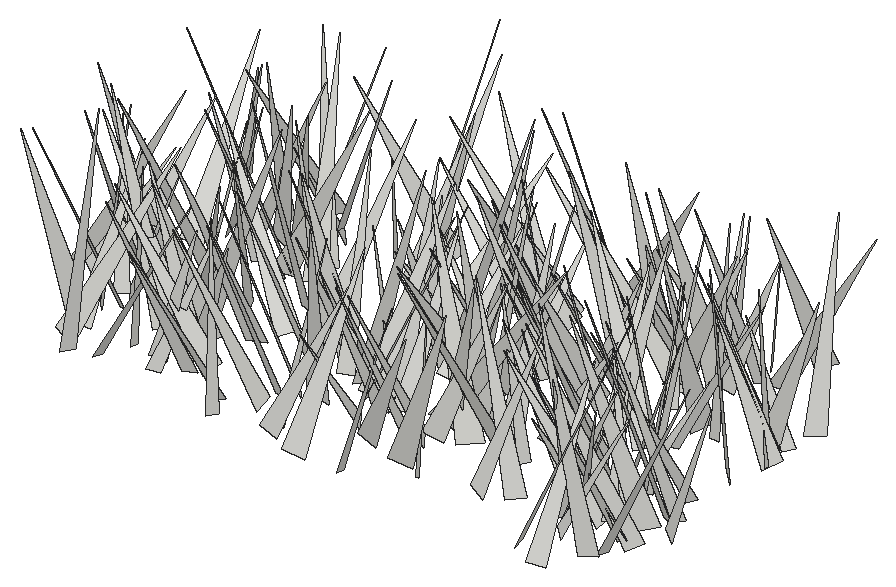
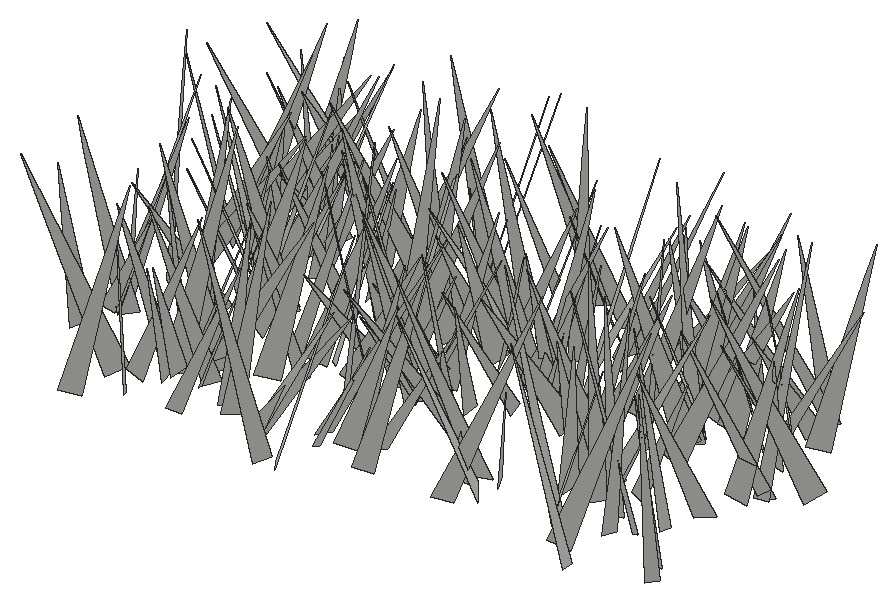
# SketchUp Ruby script. Lengths in inches.
U = 1.inch
M = Sketchup.active_model
def pt(a) = Geom::Point3d.new(a.map { |v| v * U })
def face(e, loops, mat)
  f = e.add_face(loops[0].map { |a| pt(a) })
  loops[1..].each { |l| e.add_face(l.map { |a| pt(a) }).erase! }
  f.material = f.back_material = mat if mat
  f
end
# faces: each face lists its corners as indices into pts; further lists are holes
def faces(e, pts, list, mat = nil) = list.each { |f| face(e, (f[0].is_a?(Array) ? f : [f]).map { |l| l.map { |i| pts[i] } }, mat) }
# xy, xz, yz: faces in a plane at the given z, y or x. An outline is a flat list of corners, or four numbers for a rectangle; further outlines are holes
def ring(l) = l.size == 4 ? [[l[0], l[1]], [l[2], l[1]], [l[2], l[3]], [l[0], l[3]]] : l.each_slice(2).to_a
def flat(e, list, mat, &to3) = list.each { |f| face(e, (f[0].is_a?(Array) ? f : [f]).map { |l| ring(l).map { |u, v| to3.(u, v) } }, mat) }
def xy(e, z, list, mat = nil) = flat(e, list, mat) { |x, y| [x, y, z] }
def xz(e, y, list, mat = nil) = flat(e, list, mat) { |x, z| [x, y, z] }
def yz(e, x, list, mat = nil) = flat(e, list, mat) { |y, z| [x, y, z] }
def lines(e, pts, list) = list.each { |a, b| e.add_line(pt(pts[a]), pt(pts[b])) }
# prism: a flat outline (further loops are holes) pulled along v
def prism(e, loops, v, mat = nil)
  f = face(e, loops, mat); d = Geom::Vector3d.new(v.map { |x| x * U })
  f.pushpull(f.normal.samedirection?(d) ? d.length : -d.length)
end
def box(e, o, s, mat = nil) = prism(e, [[o, [o[0] + s[0], o[1], o[2]], [o[0] + s[0], o[1] + s[1], o[2]], [o[0], o[1] + s[1], o[2]]]], [0, 0, s[2]], mat)
def at(x, y, z, deg = 0) = Geom::Transformation.translation(pt([x, y, z])) * Geom::Transformation.rotation(ORIGIN, Z_AXIS, deg.degrees)
def axes(o, x, y, z) = Geom::Transformation.new([*x, 0, *y, 0, *z, 0, *pt(o).to_a, 1])
def part(name) = M.definitions.add(name)
# library, detail: a bought-in or finely detailed component or shape, given as its bounding box
def library(name, o, s) = part(name).tap { |d| box(d.entities, o, s) }
def detail(e, o, s) = box(e.add_group.entities, o, s)
def put(e, d, t, mat = nil) = e.add_instance(d, t).tap { |i| i.material = mat if mat }
def group(e, t, mat = nil) = e.add_group.tap { |g| g.transformation = t; g.material = mat if mat }.entities
root = M.entities
c1 = part("fur_instance\#9")
p = [[0.8125,0,1.79],[0.67,-0.02,1.48],[0,-0.11,0],[0,0.11,0]]
faces(c1.entities,p,[[0,1,2,3]])
put(root,c1,axes([523.85,208.09,-21.66],[-1.22058,7.14872,1.6543],[7.02907,1.62036,-1.81584],[2.10547,-1.26529,7.02116]))
put(root,c1,axes([518.5,211.77,-21.66],[-6.87561,-0.89332,0.66489],[-0.69538,6.69239,1.80069],[0.86979,-1.71115,6.69549]))
put(root,c1,axes([529.6875,211.27,-21.66],[2.97269,-7.01093,0.81561],[-6.80259,-2.60982,2.35986],[1.88234,1.64042,7.24024]))
put(root,c1,axes([520.92,209.3125,-21.66],[0.63179,6.0642,2.01169],[5.81387,0.29266,-2.70812],[2.6496,-2.08816,5.46258]))
put(root,c1,axes([516.1,210.75,-21.66],[-2.43401,-4.94438,0.27236],[-4.40728,2.02468,-2.63096],[-2.25763,1.37813,4.84245]))
put(root,c1,axes([527.43,208.23,-21.66],[5.0446,1.96996,1.21492],[1.59207,-5.06819,1.60732],[-1.6799,1.1124,5.17158]))
put(root,c1,axes([545.87,209.39,-21.66],[-0.49595,7.7495,2.67586],[7.77568,-0.40515,2.61451],[-2.59882,-2.6911,7.31198]))
put(root,c1,axes([544.01,206.62,-21.66],[-5.33853,3.8285,0.2094],[3.37353,4.86067,-2.86257],[1.82225,2.21756,5.91295]))
put(root,c1,axes([526.25,212.25,-21.66],[0.97454,-6.53217,0.4424],[-5.83998,-0.6651,3.04417],[2.95966,0.83851,5.86106]))
put(root,c1,axes([529.08,213.2,-21.66],[-5.93761,-4.29126,0.84113],[-3.95201,5.87307,2.0655],[1.8719,-1.21235,7.02879]))
put(root,c1,axes([512.45,212.18,-21.66],[-0.7364,-6.55979,0.93298],[-6.36781,0.44127,-1.92351],[-1.83094,1.10364,6.31453]))
put(root,c1,axes([541.55,207.9375,-21.66],[7.40987,3.38689,0.1989],[3.26816,-7.25381,1.76579],[-0.91088,1.52574,7.95356]))
put(root,c1,axes([516.89,208.84,-21.66],[-6.05954,0.33778,0.89505],[0.02694,5.79744,-2.00555],[0.95629,1.97708,5.728]))
put(root,c1,axes([542.67,210.61,-21.66],[3.6305,3.98779,0.322],[3.84064,-3.3521,-1.78874],[1.12055,-1.43096,5.08758]))
put(root,c1,axes([524.49,213.84,-21.66],[-4.06772,-3.26977,0.32403],[-2.78571,3.7053,2.41936],[1.74246,-1.70943,4.62433]))
put(root,c1,axes([542.39,213.06,-21.66],[6.00758,0.21792,0.49644],[0.387,-5.59183,-2.22857],[-0.3797,-2.2514,5.58318]))
put(root,c1,axes([528.79,214.74,-21.66],[-5.78164,-4.6449,0.78576],[-4.06196,5.54542,2.89287],[2.386,-1.8147,6.82889]))
put(root,c1,axes([541.35,213.38,-21.66],[5.83634,-0.86723,1.56304],[-0.35494,-5.79341,-1.88904],[-1.75191,-1.71533,5.58985]))
put(root,c1,axes([543.97,213.47,-21.66],[-6.77007,0.71674,0.61078],[0.8862,6.3486,2.37288],[0.31848,-2.42944,6.38099]))
put(root,c1,axes([546.32,212.17,-21.66],[-2.71557,-5.16024,0.69315],[-4.67023,2.06855,-2.89705],[-2.30163,1.89099,5.06058]))
put(root,c1,axes([504.96,209.6,-21.66],[-7.30658,0.78889,2.52937],[0.00726,7.42557,-2.29501],[2.64953,2.15518,6.98151]))
put(root,c1,axes([546.38,210.21,-21.66],[6.37696,0.70596,0.43543],[0.57496,-6.19552,1.62437],[-0.59783,1.57187,6.20688]))
put(root,c1,axes([547.43,212.01,-21.66],[-2.51256,7.06983,2.10699],[6.38069,0.96553,4.36915],[-3.70253,-3.13371,6.09968]))
put(root,c1,axes([513.34,213.27,-21.66],[-6.69596,1.51903,0.23584],[1.52209,6.40398,1.96756],[-0.2152,-1.96993,6.57815]))
put(root,c1,axes([506.77,210.28,-21.66],[5.85572,0.96623,0.0245],[0.91904,-5.61274,1.69591],[-0.29926,1.66948,5.68743]))
put(root,c1,axes([509.88,212.27,-21.66],[-0.77614,4.62516,2.62163],[4.88719,1.66369,-1.48826],[2.09294,-2.16967,4.44742]))
put(root,c1,axes([502.29,213.94,-21.66],[3.31279,-6.01066,2.01721],[-5.81791,-3.7865,-1.72802],[-2.51972,0.84034,6.64203]))
put(root,c1,axes([520.625,214.47,-21.66],[0.39282,-7.92697,1.06347],[-7.86049,-0.18606,1.51663],[1.47665,1.11832,7.79044]))
put(root,c1,axes([531.56,210.57,-21.66],[2.74983,3.97442,1.3241],[3.39736,-3.04242,2.07665],[-2.45097,0.24187,4.36407]))
put(root,c1,axes([518.59,213.32,-21.66],[-2.94744,-5.34651,0.76174],[-5.29498,2.69026,-1.60576],[-1.06233,1.42484,5.89017]))
put(root,c1,axes([541.13,211.91,-21.66],[5.01849,-2.22986,0.6447],[-2.32023,-4.77497,1.54574],[0.06662,1.67347,5.26955]))
put(root,c1,axes([535.53,211.39,-21.66],[2.61038,6.20008,1.07332],[6.21386,-2.35716,-1.49626],[0.99041,-1.55238,6.55868]))
put(root,c1,axes([541.64,214.5,-21.66],[1.73038,-3.85975,0.19684],[-3.59553,-1.68683,-1.46882],[-1.41726,-0.43309,3.96667]))
put(root,c1,axes([503.67,210.87,-21.66],[1.59933,7.72158,1.03232],[7.26868,-1.09996,-3.03359],[2.80263,-1.55359,7.2786]))
put(root,c1,axes([510.63,210.89,-21.66],[-3.36626,3.2291,1.55087],[2.48228,3.63709,-2.18492],[2.58275,0.71309,4.12128]))
put(root,c1,axes([521.01,210.36,-21.66],[3.09687,5.17866,0.3937],[4.90573,-3.06729,1.75775],[-1.70508,0.58082,5.7723]))
put(root,c1,axes([546.59,214.31,-21.66],[2.25381,-7.00366,2.80187],[-6.80723,-3.14832,-2.39397],[-3.25014,1.7373,6.957]))
put(root,c1,axes([534.25,216.01,-21.66],[-1.51333,-7.7582,0.0595],[-7.60064,1.47034,-1.59746],[-1.5568,0.36304,7.74132]))
put(root,c1,axes([537.9375,212.27,-21.66],[-2.07893,6.71015,1.41675],[6.64432,1.60395,2.15305],[-1.69892,-1.93817,6.68674]))
put(root,c1,axes([511.91,213.58,-21.66],[2.26565,-5.57265,3.25786],[-5.77256,-3.29433,-1.62055],[-2.88887,2.21229,5.79322]))
put(root,c1,axes([511,214.83,-21.66],[2.55159,-4.81811,0.15811],[-4.66384,-2.42197,1.46026],[1.21971,0.81832,5.25284]))
put(root,c1,axes([519.61,214.1,-21.66],[-5.18196,-4.15409,0.26027],[-4.02731,4.89921,-1.98883],[-1.05116,1.70828,6.3367]))
put(root,c1,axes([548.17,214.39,-21.66],[3.55889,4.26793,1.49162],[4.48448,-3.09137,-1.85436],[0.57409,-2.30955,5.23854]))
put(root,c1,axes([507.77,212.61,-21.66],[-5.27031,-0.93158,1.82448],[-1.52104,5.15288,-1.7627],[1.37223,2.13373,5.05341]))
put(root,c1,axes([542.1,211.6,-21.66],[3.66299,2.22216,0.32756],[1.7102,-3.16536,2.34915],[-1.4562,1.87225,3.58288]))
put(root,c1,axes([511.16,216.47,-21.66],[3.93068,-5.30389,1.53813],[-4.85639,-4.21869,-2.1367],[-2.62918,-0.13704,6.24628]))
put(root,c1,axes([524.76,215.58,-21.66],[-0.6126,-5.21006,0.97224],[-5.10965,0.32064,-1.50131],[-1.40764,1.1035,5.02654]))
put(root,c1,axes([529.17,216.78,-21.66],[-0.1774,-7.7519,1.13116],[-7.17611,0.61466,3.08685],[3.14245,0.96602,7.113]))
put(root,c1,axes([517.81,217.43,-21.66],[-5.57338,-5.53642,0.81265],[-5.27737,5.58191,1.83481],[1.86058,-0.75178,7.63858]))
put(root,c1,axes([540.28,215.0625,-21.66],[-4.33976,4.07233,1.17149],[4.17045,3.80756,2.21352],[-0.75076,-2.38923,5.52429]))
put(root,c1,axes([539.65,216.52,-21.66],[4.21418,-1.38432,0.79636],[-0.98829,-4.02576,-1.76817],[-1.25452,-1.47878,4.06808]))
put(root,c1,axes([541.1875,213.48,-21.66],[-1.53438,4.71255,0.03454],[4.47921,1.44703,1.55125],[-1.46492,-0.51147,4.70702]))
put(root,c1,axes([504.28,215.79,-21.66],[-3.99389,-5.07881,0.29207],[-4.86869,3.70838,-2.09153],[-1.47493,1.51142,6.11318]))
put(root,c1,axes([508.62,218.04,-21.66],[8.12463,-0.31909,0.21051],[-0.21684,-7.53553,-3.0536],[-0.31483,-3.04462,7.53571]))
put(root,c1,axes([546.88,215.91,-21.66],[-4.74845,-6.02691,1.04144],[-6.05438,4.44477,-1.88271],[-0.8676,1.96887,7.4382]))
put(root,c1,axes([513.31,217.68,-21.66],[0.28426,-7.43419,0.75555],[-7.30944,-0.43371,-1.51752],[-1.55247,0.68085,7.28321]))
put(root,c1,axes([542.23,216.57,-21.66],[-3.30387,-7.05223,0.96215],[-6.92829,2.9435,-2.21582],[-1.63048,1.78244,7.4659]))
put(root,c1,axes([529.21,215.05,-21.66],[3.36914,-5.54095,2.01408],[-5.73384,-2.5398,2.60427],[1.37175,2.99283,5.93894]))
put(root,c1,axes([545.06,214.375,-21.66],[-1.00856,5.27208,0.80529],[5.17147,0.76643,1.45913],[-1.30357,-1.0384,5.16556]))
put(root,c1,axes([544.16,213.5625,-21.66],[-4.2837,1.86088,0.37109],[1.60299,4.03921,-1.75094],[1.01537,1.47394,4.32979]))
put(root,c1,axes([507.96,215.45,-21.66],[-2.53782,7.33959,2.16761],[7.45924,1.86167,2.42953],[-1.71111,-2.77006,7.37615]))
put(root,c1,axes([503.67,212.53,-21.66],[-4.95607,3.58078,0.35964],[3.00453,4.45388,-2.94106],[1.98095,2.2034,5.36049]))
put(root,c1,axes([509.98,214.94,-21.66],[-2.8355,7.09509,0.7949],[6.33308,2.10473,3.80453],[-3.2961,-2.05963,6.62616]))
put(root,c1,axes([531.46,215.89,-21.66],[-4.16616,6.68617,2.08588],[7.00105,3.90518,1.46546],[-0.20279,-2.54114,7.74043]))
put(root,c1,axes([539.29,219.57,-21.66],[-6.65977,-5.09555,0.25994],[-4.96209,6.56797,1.61994],[1.1874,-1.13219,8.22757]))
put(root,c1,axes([547.53,216.24,-21.66],[-2.26256,-5.81888,2.33683],[-5.71547,0.89178,-3.31322],[-2.57945,3.12805,5.2916]))
put(root,c1,axes([503.11,215.1875,-21.66],[4.45887,4.52554,1.75159],[4.30275,-4.78695,1.41478],[-2.24387,-0.18639,6.19358]))
put(root,c1,axes([503.71,217.19,-21.66],[4.52674,3.32324,0.78926],[3.39525,-4.2348,-1.64226],[0.37301,-1.78348,5.37013]))
put(root,c1,axes([529.09,221.12,-21.66],[4.10096,-6.21113,0.1393],[-5.64172,-3.79303,-3.03306],[-2.60165,-1.56533,6.79681]))
put(root,c1,axes([528.28,217.11,-21.66],[5.80573,-6.03364,0.3689],[-5.4436,-4.99608,3.95649],[2.62833,2.98023,7.37953]))
put(root,c1,axes([519.07,219.81,-21.66],[-5.21619,-2.22313,1.39253],[-1.54183,5.10575,2.37575],[2.12232,-1.75473,5.14847]))
put(root,c1,axes([535.4,219.18,-21.66],[-3.59225,-3.71334,1.0598],[-3.39845,3.72735,1.54069],[1.83374,-0.36648,4.93148]))
put(root,c1,axes([535.61,216,-21.66],[-5.65883,0.17912,0.29432],[0.09895,5.4838,-1.43499],[0.33003,1.4272,5.47679]))
put(root,c1,axes([501.11,221.01,-21.66],[-2.73458,-7.67612,0.26637],[-7.34259,2.69559,2.30041],[2.25392,-0.53168,7.81722]))
put(root,c1,axes([530.47,219.11,-21.66],[6.98287,-2.99298,2.96369],[-2.61118,-7.57832,-1.50091],[-3.30502,-0.33623,7.44753]))
put(root,c1,axes([542.3,217.4,-21.66],[-6.0406,-4.0795,1.11122],[-4.22494,5.74856,-1.86274],[-0.16426,2.16279,7.04708]))
put(root,c1,axes([519.375,219.46,-21.66],[4.80769,-4.80499,2.60276],[-4.52111,-5.44469,-1.70033],[-3.0695,0.49361,6.58109]))
put(root,c1,axes([546.54,218.74,-21.66],[-1.84266,-5.86998,0.99209],[-5.21002,1.08759,-3.24178],[-2.88039,1.78795,5.22904]))
put(root,c1,axes([541.58,219.09,-21.66],[6.21728,1.67139,0.47713],[1.73743,-6.02723,-1.52629],[-0.05031,-1.59834,6.25448]))
put(root,c1,axes([521.3,218.96,-21.66],[-4.03956,-5.75099,0.92293],[-5.66396,3.6166,-2.25467],[-1.3584,2.0224,6.65646]))
put(root,c1,axes([508.27,220.7,-21.66],[-1.35129,-7.71927,0.81651],[-7.46816,1.06686,-2.27338],[-2.11671,1.16382,7.49966]))
put(root,c1,axes([510.46,220.51,-21.66],[5.99792,1.55177,2.60045],[2.40829,-5.94226,-2.00876],[-1.83589,-2.72525,5.86071]))
put(root,c1,axes([521.625,217.77,-21.66],[7.44072,-1.6859,2.03296],[-2.09272,-7.4711,1.46382],[-1.61112,1.91833,7.48758]))
put(root,c1,axes([522.96,216.68,-21.66],[-0.55252,7.61083,1.2014],[7.43516,0.84266,-1.91879],[2.02152,-1.01911,7.38568]))
put(root,c1,axes([524.03,217.79,-21.66],[-5.16392,-1.1559,0.80889],[-1.35151,4.93357,-1.57791],[0.40477,1.72635,5.05098]))
put(root,c1,axes([535,218.875,-21.66],[2.54302,-4.52945,1.06711],[-4.23804,-1.75205,2.66287],[1.92189,2.12978,4.46004]))
put(root,c1,axes([533.24,217.39,-21.66],[5.43285,-3.6045,3.64876],[-4.74936,-5.54221,1.59663],[-1.93634,3.48041,6.32132]))
put(root,c1,axes([503.06,217.26,-21.66],[-0.43332,5.55714,0.38235],[5.39105,0.32188,1.43136],[-1.40165,-0.47995,5.3871]))
put(root,c1,axes([508.75,218.6,-21.66],[6.76451,-3.26106,1.25254],[-3.47694,-6.54929,1.72622],[-0.33809,2.1058,7.30844]))
put(root,c1,axes([522.96,216.33,-21.66],[6.18332,3.30926,0.01495],[3.17233,-5.93637,1.96995],[-0.9422,1.73008,6.73082]))
put(root,c1,axes([509.18,216.54,-21.66],[4.35483,5.04158,0.80125],[4.65214,-4.35304,2.10539],[-2.1017,0.81089,6.32055]))
put(root,c1,axes([525.7,216.42,-21.66],[-4.59878,4.14257,0.47856],[3.69105,4.37512,-2.40275],[1.94062,1.49539,5.70408]))
put(root,c1,axes([499.58,218.4,-21.66],[2.70061,4.81345,0.08968],[4.52857,-2.505,-1.92033],[1.63383,-1.01307,5.17446]))
put(root,c1,axes([543.93,217.32,-21.66],[4.5947,4.98178,1.41698],[4.55399,-4.78808,2.06705],[-2.46722,0.43974,6.4542]))
put(root,c1,axes([527.27,224.41,-21.66],[-5.00279,-6.48805,0.18943],[-5.66686,4.48249,3.86684],[3.16501,-2.22958,7.22289]))
put(root,c1,axes([498.68,218.8,-21.66],[6.56364,-3.25708,1.01889],[-3.38805,-5.95385,2.79299],[0.40967,2.94467,6.77415]))
put(root,c1,axes([502.38,221.97,-21.66],[0.14854,-7.36709,1.66817],[-7.40985,-0.46607,-1.39849],[-1.46661,1.60862,7.23466]))
put(root,c1,axes([542.14,220.1875,-21.66],[2.38056,3.51502,0.37387],[3.33138,-2.08023,-1.65431],[1.18197,-1.21634,3.90969]))
put(root,c1,axes([514.18,219.66,-21.66],[-4.44973,5.42889,0.1833],[5.21151,4.19987,2.12315],[-1.53186,-1.48148,6.69068]))
put(root,c1,axes([524.9,222.13,-21.66],[2.07945,-5.56592,1.40736],[-5.43571,-2.39045,-1.42237],[-1.84751,0.76846,5.76892]))
put(root,c1,axes([520.09,217.88,-21.66],[0.51601,7.02264,0.2402],[6.84431,-0.55684,1.57697],[-1.5908,-0.11784,6.86272]))
put(root,c1,axes([528.64,222.16,-21.66],[2.77166,-6.45652,0.14972],[-5.9267,-2.47813,2.8503],[2.56578,1.25036,6.42219]))
put(root,c1,axes([524.51,217.58,-21.66],[-6.77077,3.15469,0.89527],[2.64884,6.47215,-2.77341],[1.93319,2.18084,6.93567]))
put(root,c1,axes([546.23,222.625,-21.66],[-5.2101,-5.93708,2.74108],[-5.84341,5.80017,1.45611],[2.93548,1.00834,7.76362]))
put(root,c1,axes([532.09,224.05,-21.66],[-3.9218,-4.42687,0.35438],[-4.07666,3.77609,2.05553],[1.7617,-1.11678,5.54549]))
put(root,c1,axes([516.67,220.09,-21.66],[-7.00273,-0.39667,0.95685],[-0.59042,6.90153,-1.45992],[0.85107,1.52402,6.86034]))
put(root,c1,axes([542.36,220.85,-21.66],[-3.42492,-4.02626,1.68032],[-4.34426,2.9504,-1.78518],[-0.40205,2.41841,4.97534]))
put(root,c1,axes([530.37,218.93,-21.66],[3.83849,6.3713,1.10198],[6.13828,-3.99344,1.70758],[-2.03209,-0.02789,7.23959]))
put(root,c1,axes([534.58,224.9,-21.66],[-6.04066,-0.63869,2.51357],[0.73038,5.69455,3.20222],[2.48847,-3.22176,5.16172]))
put(root,c1,axes([538.41,220.74,-21.66],[-1.59502,6.99566,2.35908],[7.02793,2.17795,-1.70682],[2.26111,-1.83463,6.96922]))
put(root,c1,axes([525,224.38,-21.66],[-5.02387,-1.18033,0.42976],[-0.88594,4.58548,2.23734],[0.8905,-2.09699,4.65046]))
put(root,c1,axes([538.34,223.8,-21.66],[-2.23247,-5.83337,0.18602],[-5.6892,2.13065,-1.46288],[-1.30221,0.692,6.07224]))
put(root,c1,axes([543.93,217.75,-21.66],[4.35175,7.0169,0.44581],[6.16578,-4.0605,3.72408],[-3.37917,1.6275,7.36925]))
put(root,c1,axes([500.89,220.7,-21.66],[0.65701,6.39206,0.99008],[6.12037,-0.29236,-2.17392],[2.09278,-1.15171,6.04683]))
put(root,c1,axes([533.23,224.59,-21.66],[1.95168,-6.84621,1.26966],[-6.52036,-2.2596,-2.16121],[-2.44285,0.56154,6.78298]))
put(root,c1,axes([513.05,222.8,-21.66],[-3.81075,-5.76969,1.72606],[-6.01138,3.52106,-1.50194],[-0.36316,2.25903,6.74947]))
put(root,c1,axes([540.23,222.14,-21.66],[-4.97351,5.86998,1.15657],[5.9442,4.67754,1.82131],[-0.6788,-2.04794,7.47498]))
put(root,c1,axes([538.38,220.56,-21.66],[-4.13598,4.27474,0.09369],[4.07434,3.97972,-1.71759],[1.29691,1.13001,5.6947]))
put(root,c1,axes([519.9,221.63,-21.66],[4.92859,0.75105,0.39032],[0.57555,-4.66461,1.7081],[-0.62062,1.63853,4.68375]))
put(root,c1,axes([541.375,226.27,-21.66],[6.17469,-3.94346,0.96595],[-3.5616,-6.10514,-2.15707],[-1.94909,-1.33681,7.00177]))
put(root,c1,axes([527.08,223.87,-21.66],[-3.88127,2.88585,0.74535],[2.95869,3.58243,1.53633],[-0.36036,-1.66913,4.58608]))
put(root,c1,axes([509.43,224.89,-21.66],[-2.97,-5.19915,0.68344],[-5.09037,2.66981,-1.8109],[-1.25951,1.46972,5.70725]))
put(root,c1,axes([547.59,225.29,-21.66],[-5.95975,2.47486,1.75961],[2.91321,5.75356,1.77469],[0.85695,-2.34763,6.20435]))
put(root,c1,axes([546.71,227.02,-21.66],[-5.73536,-5.62008,0.65862],[-5.46135,5.74328,1.44982],[1.48081,-0.58562,7.89796]))
put(root,c1,axes([525.1,221.43,-21.66],[-2.44099,4.81015,0.04297],[4.37742,2.2412,-2.21652],[1.99437,0.96814,4.91762]))
put(root,c1,axes([521.98,223.43,-21.66],[-4.57761,1.25738,1.06742],[0.91701,4.55759,-1.43608],[1.37093,1.14988,4.52473]))
put(root,c1,axes([528.41,227.64,-21.66],[-4.91582,-6.36103,2.07601],[-5.8042,5.33544,2.60426],[3.32923,-0.09063,7.60565]))
put(root,c1,axes([515.68,221.44,-21.66],[-5.17652,4.83446,1.05401],[3.91261,4.93311,-3.41105],[3.02894,1.88989,6.20751]))
put(root,c1,axes([527.79,225.81,-21.66],[5.79589,4.16761,1.50359],[4.42839,-5.37215,-2.17978],[0.13803,-2.64446,6.79779]))
put(root,c1,axes([508.77,227.38,-21.66],[7.2919,-1.58164,0.56037],[-1.39543,-7.10365,-1.89164],[-0.93186,-1.73896,7.21769]))
put(root,c1,axes([541.37,223.19,-21.66],[5.52796,-0.81869,0.7417],[-1.07099,-4.89962,2.57397],[-0.27083,2.66498,4.96017]))
put(root,c1,axes([530.12,225.22,-21.66],[-1.81659,5.58818,1.87966],[5.39696,0.78429,2.88421],[-2.37355,-2.49359,5.11948]))
put(root,c1,axes([509.28,225.83,-21.66],[-6.03257,-5.76703,0.56772],[-5.59645,5.58532,-2.7307],[-1.50355,2.34912,7.8863]))
put(root,c1,axes([509.28,225.32,-21.66],[5.54301,-4.89223,1.08245],[-4.92161,-5.01325,2.54471],[0.93987,2.60075,6.94141]))
put(root,c1,axes([529.46,222.76,-21.66],[-3.68567,4.23937,0.30212],[3.60627,3.33103,-2.74713],[2.24908,1.60613,4.89997]))
put(root,c1,axes([507.11,225.59,-21.66],[-0.49335,5.1966,1.87912],[5.02115,-0.36617,2.33091],[-2.30734,-1.90798,4.67065]))
put(root,c1,axes([524.16,223.25,-21.66],[7.79418,1.63756,2.08164],[0.8535,-7.67768,2.8441],[-2.50726,2.47704,7.43922]))
put(root,c1,axes([547.46,225.0625,-21.66],[-5.30333,-1.20318,1.41609],[-1.56427,5.2022,-1.4382],[1.00301,1.75149,5.24448]))
put(root,c1,axes([503.37,227.57,-21.66],[6.27835,0.76334,0.54412],[0.88551,-6.03847,-1.74618],[-0.30762,-1.80294,6.07875]))
put(root,c1,axes([506.75,228.24,-21.66],[-0.2881,-6.79413,1.19024],[-6.52945,0.65262,2.14482],[2.22333,1.03623,6.45314]))
put(root,c1,axes([532.37,226.8,-21.66],[1.52627,-4.48364,1.33128],[-4.39877,-0.90019,2.01128],[1.58937,1.81423,4.28804]))
put(root,c1,axes([545.87,227.02,-21.66],[3.29636,-5.4576,1.30622],[-5.51274,-2.86598,1.93739],[1.04942,2.08768,6.07437]))
put(root,c1,axes([525.49,224.66,-21.66],[-6.79191,0.51616,3.38033],[-0.49773,7.28774,-2.11287],[3.3831,2.10844,6.47551]))
put(root,c1,axes([534.21,228,-21.66],[4.0303,-5.81988,3.12764],[-5.66664,-4.92868,-1.86917],[-3.39741,1.31665,6.82792]))
put(root,c1,axes([525.58,224.1,-21.66],[4.27823,3.00126,0.70858],[2.21616,-3.83495,2.86263],[-2.14435,2.02448,4.3722]))
put(root,c1,axes([547.22,227.37,-21.66],[-1.85647,3.95367,0.8299],[3.82368,1.42492,1.76516],[-1.30372,-1.4508,3.99527]))
put(root,c1,axes([542.79,225.58,-21.66],[2.80201,6.02167,1.40008],[5.6342,-3.12002,2.14317],[-2.54489,-0.27744,6.28638]))
put(root,c1,axes([502.4,224.87,-21.66],[-2.48989,6.58556,0.19317],[6.42005,2.47161,-1.51018],[1.47984,0.3578,6.87667]))
put(root,c1,axes([536.97,229,-21.66],[3.33833,-6.51025,0.54896],[-6.14625,-2.92038,2.74304],[2.21549,1.70799,6.78259]))
put(root,c1,axes([537.54,228.91,-21.66],[-4.43221,4.72995,1.58971],[4.78005,3.41433,3.16821],[-1.43205,-3.24253,5.65503]))
put(root,c1,axes([504.45,229.17,-21.66],[5.46808,5.3055,1.78388],[5.41419,-4.38056,-3.56761],[1.42026,-3.72732,6.73205]))
put(root,c1,axes([505.75,230.11,-21.66],[6.82649,-0.20783,2.36031],[0.47416,-6.93274,-1.9818],[-2.32152,-2.02711,6.5358]))
put(root,c1,axes([524.76,231.03,-21.66],[3.41213,-4.67618,0.33772],[-4.46229,-3.36731,-1.54031],[-1.43828,-0.64649,5.58003]))
put(root,c1,axes([539.12,230.97,-21.66],[5.28612,-6.00356,2.19792],[-5.60526,-5.72373,-2.15328],[-3.07484,0.113,7.70384]))
put(root,c1,axes([536.71,231.47,-21.66],[-4.92711,-3.11526,0.5387],[-2.69685,4.66208,2.29422],[1.64986,-1.68274,5.3589]))
put(root,c1,axes([509.4375,231.15,-21.66],[-3.6044,-3.37024,0.34721],[-3.01204,3.4196,1.92476],[1.55135,-1.19103,4.54373]))
put(root,c1,axes([538.32,226.93,-21.66],[-4.43133,1.84787,0.51045],[1.62369,4.30117,-1.47494],[1.01922,1.18203,4.56901]))
put(root,c1,axes([521.04,225.91,-21.66],[-1.51427,6.54379,0.36236],[5.84338,1.51647,-2.96661],[2.96773,0.35306,6.02606]))
put(root,c1,axes([511.43,225.76,-21.66],[-6.67493,4.02137,0.12146],[3.83511,6.43107,-2.16198],[1.21576,1.79188,7.48679]))
put(root,c1,axes([527.21,231.26,-21.66],[-8.16776,0.06376,0.0825],[0.08376,7.86119,2.21763],[0.06209,-2.2183,7.8612]))
put(root,c1,axes([539.56,228.27,-21.66],[-6.70794,-1.60484,0.19836],[-1.59675,6.44001,-1.8942],[-0.25542,1.88735,6.63204]))
put(root,c1,axes([508.95,231.11,-21.66],[8.07507,1.50255,0.4439],[1.56674,-7.73574,-2.31627],[0.00564,-2.35841,7.88031]))
put(root,c1,axes([522.47,233.33,-21.66],[4.86562,-4.5964,0.06859],[-4.19123,-4.47675,-2.68294],[-1.88818,-1.90726,6.13213]))
put(root,c1,axes([507.2,233.21,-21.66],[2.70234,-6.75975,0.1599],[-6.39067,-2.60962,-2.31767],[-2.20886,-0.71979,6.90111]))
put(root,c1,axes([511.02,227.54,-21.66],[-7.30125,2.0292,0.54339],[1.84392,7.1322,-1.85816],[1.00641,1.65384,7.34664]))
put(root,c1,axes([533.92,232.22,-21.66],[4.85347,-3.26157,0.26621],[-3.0891,-4.72355,-1.55255],[-1.07988,-1.1468,5.6377]))
put(root,c1,axes([516.47,230.67,-21.66],[3.82304,5.79974,2.60132],[6.29108,-3.01834,-2.51622],[0.9089,-3.50316,6.47466]))
put(root,c1,axes([523.32,230.64,-21.66],[-5.14523,1.96025,0.06602],[1.88898,4.90265,1.64806],[-0.52792,-1.56261,5.25356]))
put(root,c1,axes([514.91,229.35,-21.66],[-3.90269,-1.36809,1.23152],[-1.73858,3.68797,-1.41263],[0.60468,1.77384,3.88679]))
put(root,c1,axes([536.375,230.65,-21.66],[2.73482,-5.11249,1.4467],[-5.08402,-2.04521,2.38319],[1.54377,2.32148,5.28557]))
put(root,c1,axes([516.375,233.2,-21.66],[-6.66712,2.68909,2.42043],[3.53397,5.92752,3.14894],[0.77508,-3.89533,6.46266]))
put(root,c1,axes([500.76,231.53,-21.66],[-1.89095,-4.65132,2.366],[-4.60338,2.67208,1.57395],[2.45798,1.42605,4.76793]))
put(root,c1,axes([539.4,230.84,-21.66],[-0.77235,4.89048,2.70767],[4.92537,1.88806,-2.00519],[2.64368,-2.08884,4.52687]))
put(root,c1,axes([526.59,232.74,-21.66],[-3.56897,-0.50146,0.42511],[-0.28446,3.29362,1.49696],[0.59267,-1.43888,3.27843]))
put(root,c1,axes([533.05,232.84,-21.66],[-6.0404,2.2493,3.21945],[3.13358,6.3206,1.46334],[2.36747,-2.62704,6.2773]))
put(root,c1,axes([499.96,233.15,-21.66],[5.73315,-1.08828,0.33068],[-0.98004,-5.58896,-1.40205],[-0.57725,-1.3198,5.66459]))
put(root,c1,axes([516.2,229.52,-21.66],[0.38295,8.08113,1.09098],[7.9956,-0.1576,-1.6392],[1.60161,-1.14545,7.92239]))
put(root,c1,axes([547.3125,229.82,-21.66],[-5.92088,3.75972,1.43779],[3.50525,6.07307,-1.44586],[1.97886,0.49178,6.86307]))
put(root,c1,axes([540.71,232.85,-21.66],[-1.01411,-6.0227,1.51425],[-5.97973,0.53295,-1.88497],[-1.67593,1.7428,5.80932]))
put(root,c1,axes([536.11,234.8,-21.66],[3.38656,-3.48151,1.0277],[-2.77448,-3.38882,-2.33752],[-2.3408,-1.02022,4.25743]))
put(root,c1,axes([525.11,231.69,-21.66],[-3.78872,6.01371,0.63065],[5.87535,3.48538,2.06137],[-1.42923,-1.61377,6.8022]))
put(root,c1,axes([530.73,233.27,-21.66],[-3.83855,4.56526,0.77541],[4.17711,2.97899,3.13921],[-1.99865,-2.54191,5.07163]))
put(root,c1,axes([538.84,230.88,-21.66],[-5.03448,1.97141,0.87824],[1.57247,4.87743,-1.93439],[1.47821,1.52579,5.04882]))
put(root,c1,axes([541.9,233.07,-21.66],[6.07863,-4.42165,0.21276],[-4.21796,-5.67554,2.55792],[1.3435,2.18706,7.06807]))
put(root,c1,axes([539.06,231.73,-21.66],[-5.01986,0.40192,1.5189],[-0.17545,4.90978,-1.87904],[1.56135,1.84392,4.67223]))
put(root,c1,axes([526.98,236.28,-21.66],[-6.21102,-4.85766,0.88936],[-4.64444,6.23147,1.60082],[1.67841,-0.73247,7.72082]))
put(root,c1,axes([539.78,235,-21.66],[4.17117,1.8451,1.43695],[2.27213,-3.89306,-1.59669],[-0.55375,-2.07548,4.27243]))
put(root,c1,axes([530.96,232.54,-21.66],[-6.11447,-3.98639,0.59028],[-3.68819,5.10346,-3.73879],[-1.62389,3.41906,6.26894]))
put(root,c1,axes([505.19,234.93,-21.66],[6.89965,2.05968,0.48381],[2.11498,-6.67017,-1.76557],[0.05673,-1.82978,6.98071]))
put(root,c1,axes([528.01,236.26,-21.66],[1.13503,-7.67663,0.6742],[-6.50823,-0.58999,4.2389],[4.12651,1.18099,6.50005]))
put(root,c1,axes([515.25,231.12,-21.66],[6.25178,5.32919,0.93445],[4.93149,-6.20008,2.36594],[-2.22574,1.23164,7.86685]))
put(root,c1,axes([542.48,237.03,-21.66],[3.73251,-5.71066,0.85994],[-5.41751,-3.81707,-1.83396],[-2.00044,-0.31799,6.57114]))
